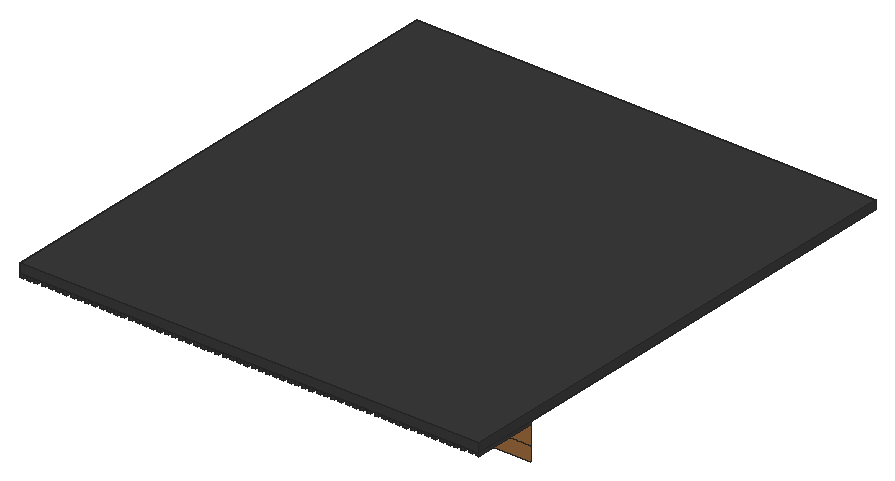
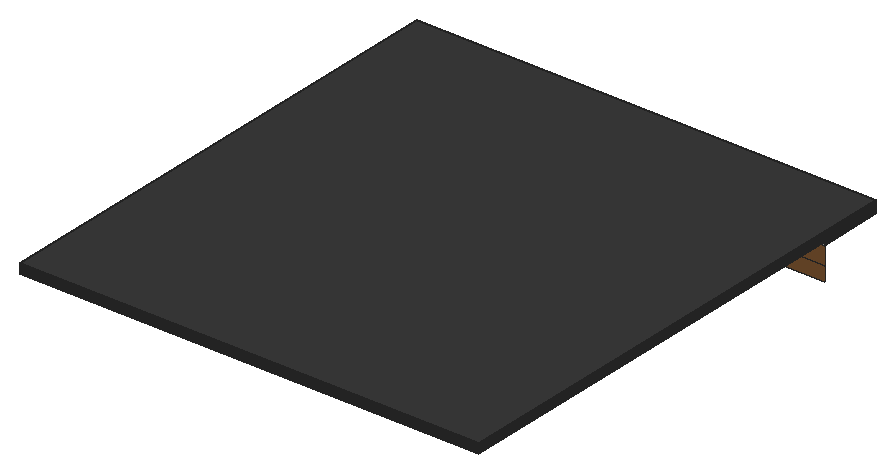
# SketchUp Ruby script. Lengths in inches.
U = 1.inch
M = Sketchup.active_model
def pt(a) = Geom::Point3d.new(a.map { |v| v * U })
def face(e, loops, mat)
  f = e.add_face(loops[0].map { |a| pt(a) })
  loops[1..].each { |l| e.add_face(l.map { |a| pt(a) }).erase! }
  f.material = f.back_material = mat if mat
  f
end
# faces: each face lists its corners as indices into pts; further lists are holes
def faces(e, pts, list, mat = nil) = list.each { |f| face(e, (f[0].is_a?(Array) ? f : [f]).map { |l| l.map { |i| pts[i] } }, mat) }
# xy, xz, yz: faces in a plane at the given z, y or x. An outline is a flat list of corners, or four numbers for a rectangle; further outlines are holes
def ring(l) = l.size == 4 ? [[l[0], l[1]], [l[2], l[1]], [l[2], l[3]], [l[0], l[3]]] : l.each_slice(2).to_a
def flat(e, list, mat, &to3) = list.each { |f| face(e, (f[0].is_a?(Array) ? f : [f]).map { |l| ring(l).map { |u, v| to3.(u, v) } }, mat) }
def xy(e, z, list, mat = nil) = flat(e, list, mat) { |x, y| [x, y, z] }
def xz(e, y, list, mat = nil) = flat(e, list, mat) { |x, z| [x, y, z] }
def yz(e, x, list, mat = nil) = flat(e, list, mat) { |y, z| [x, y, z] }
def lines(e, pts, list) = list.each { |a, b| e.add_line(pt(pts[a]), pt(pts[b])) }
# prism: a flat outline (further loops are holes) pulled along v
def prism(e, loops, v, mat = nil)
  f = face(e, loops, mat); d = Geom::Vector3d.new(v.map { |x| x * U })
  f.pushpull(f.normal.samedirection?(d) ? d.length : -d.length)
end
def box(e, o, s, mat = nil) = prism(e, [[o, [o[0] + s[0], o[1], o[2]], [o[0] + s[0], o[1] + s[1], o[2]], [o[0], o[1] + s[1], o[2]]]], [0, 0, s[2]], mat)
def at(x, y, z, deg = 0) = Geom::Transformation.translation(pt([x, y, z])) * Geom::Transformation.rotation(ORIGIN, Z_AXIS, deg.degrees)
def axes(o, x, y, z) = Geom::Transformation.new([*x, 0, *y, 0, *z, 0, *pt(o).to_a, 1])
def part(name) = M.definitions.add(name)
# library, detail: a bought-in or finely detailed component or shape, given as its bounding box
def library(name, o, s) = part(name).tap { |d| box(d.entities, o, s) }
def detail(e, o, s) = box(e.add_group.entities, o, s)
def put(e, d, t, mat = nil) = e.add_instance(d, t).tap { |i| i.material = mat if mat }
def group(e, t, mat = nil) = e.add_group.tap { |g| g.transformation = t; g.material = mat if mat }.entities
root = M.entities
M.materials.add("[Color M07]").color = [58, 58, 58]
M.materials.add("[Wood Floor]").color = [155, 105, 61]
xy(root,660.9375,[[24,175.75,456,528]])
xy(root,663.4375,[[0,33.5625,4.18,100.625],[7.5625,33.5625,11.74,100.625],[15.125,33.5625,19.31,100.625],[22.6875,33.5625,26.87,100.625],[30.25,33.5625,34.43,100.625],
  [37.8125,33.5625,41.99,100.625],[45.375,33.5625,49.56,100.625],[52.9375,33.5625,57.12,100.625],[60.5,33.5625,64.68,100.625],[68.0625,33.5625,72.24,100.625],
  [75.625,33.5625,79.81,100.625],[83.1875,33.5625,87.37,100.625],[90.75,33.5625,94.93,100.625],[98.3125,33.5625,102.49,100.625],[105.875,33.5625,110.06,100.625],
  [113.4375,33.5625,117.62,100.625],[121,33.5625,125.18,100.625],[128.5625,33.5625,132.74,100.625],[136.125,33.5625,140.31,100.625],[143.6875,33.5625,147.87,100.625],
  [151.25,33.5625,155.43,100.625],[158.8125,33.5625,162.99,100.625],[166.375,33.5625,170.56,100.625],[173.9375,33.5625,178.12,100.625],[181.5,33.5625,185.68,100.625],
  [189.0625,33.5625,193.24,100.625],[196.625,33.5625,200.81,100.625],[204.1875,33.5625,208.37,100.625],[211.75,33.5625,215.93,100.625],[219.3125,33.5625,223.49,100.625],
  [226.875,33.5625,231.06,100.625],[234.4375,33.5625,238.62,100.625],[242,33.5625,246.18,100.625],[249.5625,33.5625,253.74,100.625],[257.125,33.5625,261.31,100.625],
  [264.6875,33.5625,268.87,100.625],[272.25,33.5625,276.43,100.625],[279.8125,33.5625,283.99,100.625],[287.375,33.5625,291.56,100.625],[294.9375,33.5625,299.12,100.625],
  [302.5,33.5625,306.68,100.625],[310.0625,33.5625,314.24,100.625]],"[Color M07]")
xy(root,663.9,[[317.625,33.5625,321.81,100.625],[325.1875,33.5625,329.37,100.625],[332.75,33.5625,336.93,100.625],[340.3125,33.5625,344.49,100.625],[347.875,33.5625,352.06,100.625],
  [355.4375,33.5625,359.62,100.625],[363,33.5625,367.18,100.625],[370.5625,33.5625,374.74,100.625],[378.125,33.5625,382.31,100.625],[385.6875,33.5625,389.87,100.625],
  [393.25,33.5625,397.43,100.625],[400.8125,33.5625,404.99,100.625],[408.375,33.5625,412.56,100.625],[415.9375,33.5625,420.12,100.625],[423.5,33.5625,427.68,100.625],
  [431.0625,33.5625,435.24,100.625],[438.625,33.5625,442.81,100.625],[446.1875,33.5625,450.37,100.625],[453.75,33.5625,457.93,100.625],[461.3125,33.5625,465.49,100.625],
  [468.875,33.5625,473.06,100.625],[476.4375,33.5625,480,100.625]],"[Color M07]")
xy(root,666.9375,[[0,33.5625,4.18,100.625],[7.5625,33.5625,11.74,100.625],[15.125,33.5625,19.31,100.625],[22.6875,33.5625,26.87,100.625],[30.25,33.5625,34.43,100.625],
  [37.8125,33.5625,41.99,100.625],[45.375,33.5625,49.56,100.625],[52.9375,33.5625,57.12,100.625],[60.5,33.5625,64.68,100.625],[68.0625,33.5625,72.24,100.625],
  [75.625,33.5625,79.81,100.625],[83.1875,33.5625,87.37,100.625],[90.75,33.5625,94.93,100.625],[98.3125,33.5625,102.49,100.625],[105.875,33.5625,110.06,100.625],
  [113.4375,33.5625,117.62,100.625],[121,33.5625,125.18,100.625],[128.5625,33.5625,132.74,100.625],[136.125,33.5625,140.31,100.625],[143.6875,33.5625,147.87,100.625],
  [151.25,33.5625,155.43,100.625],[158.8125,33.5625,162.99,100.625],[166.375,33.5625,170.56,100.625],[173.9375,33.5625,178.12,100.625],[181.5,33.5625,185.68,100.625],
  [189.0625,33.5625,193.24,100.625],[196.625,33.5625,200.81,100.625],[204.1875,33.5625,208.37,100.625],[211.75,33.5625,215.93,100.625],[219.3125,33.5625,223.49,100.625],
  [226.875,33.5625,231.06,100.625],[234.4375,33.5625,238.62,100.625],[242,33.5625,246.18,100.625],[249.5625,33.5625,253.74,100.625],[257.125,33.5625,261.31,100.625],
  [264.6875,33.5625,268.87,100.625],[272.25,33.5625,276.43,100.625],[279.8125,33.5625,283.99,100.625],[287.375,33.5625,291.56,100.625],[294.9375,33.5625,299.12,100.625],
  [302.5,33.5625,306.68,100.625],[310.0625,33.5625,314.24,100.625],[317.625,33.5625,321.81,100.625],[325.1875,33.5625,329.37,100.625],[332.75,33.5625,336.93,100.625],
  [340.3125,33.5625,344.49,100.625],[347.875,33.5625,352.06,100.625],[355.4375,33.5625,359.62,100.625],[363,33.5625,367.18,100.625],[370.5625,33.5625,374.74,100.625],
  [378.125,33.5625,382.31,100.625],[385.6875,33.5625,389.87,100.625],[393.25,33.5625,397.43,100.625],[400.8125,33.5625,404.99,100.625],[408.375,33.5625,412.56,100.625],
  [415.9375,33.5625,420.12,100.625],[423.5,33.5625,427.68,100.625],[431.0625,33.5625,435.24,100.625],[438.625,33.5625,442.81,100.625],[446.1875,33.5625,450.37,100.625],
  [453.75,33.5625,457.93,100.625],[461.3125,33.5625,465.49,100.625],[468.875,33.5625,473.06,100.625],[476.4375,33.5625,480,100.625],[0,100.625,480,552]])
xy(root,666.9375,[[4.18,33.5625,7.5625,100.625],[11.74,33.5625,15.125,100.625],[19.31,33.5625,22.6875,100.625],[26.87,33.5625,30.25,100.625],[34.43,33.5625,37.8125,100.625],
  [41.99,33.5625,45.375,100.625],[49.56,33.5625,52.9375,100.625],[57.12,33.5625,60.5,100.625],[64.68,33.5625,68.0625,100.625],[72.24,33.5625,75.625,100.625],
  [79.81,33.5625,83.1875,100.625],[87.37,33.5625,90.75,100.625],[94.93,33.5625,98.3125,100.625],[102.49,33.5625,105.875,100.625],[110.06,33.5625,113.4375,100.625],
  [117.62,33.5625,121,100.625],[125.18,33.5625,128.5625,100.625],[132.74,33.5625,136.125,100.625],[140.31,33.5625,143.6875,100.625],[147.87,33.5625,151.25,100.625],
  [155.43,33.5625,158.8125,100.625],[162.99,33.5625,166.375,100.625],[170.56,33.5625,173.9375,100.625],[178.12,33.5625,181.5,100.625],[185.68,33.5625,189.0625,100.625],
  [193.24,33.5625,196.625,100.625],[200.81,33.5625,204.1875,100.625],[208.37,33.5625,211.75,100.625],[215.93,33.5625,219.3125,100.625],[223.49,33.5625,226.875,100.625],
  [231.06,33.5625,234.4375,100.625],[238.62,33.5625,242,100.625],[246.18,33.5625,249.5625,100.625],[253.74,33.5625,257.125,100.625],[261.31,33.5625,264.6875,100.625],
  [268.87,33.5625,272.25,100.625],[276.43,33.5625,279.8125,100.625],[283.99,33.5625,287.375,100.625],[291.56,33.5625,294.9375,100.625],[299.12,33.5625,302.5,100.625],
  [306.68,33.5625,310.0625,100.625],[314.24,33.5625,317.625,100.625],[321.81,33.5625,325.1875,100.625],[329.37,33.5625,332.75,100.625],[336.93,33.5625,340.3125,100.625],
  [344.49,33.5625,347.875,100.625],[352.06,33.5625,355.4375,100.625],[359.62,33.5625,363,100.625],[367.18,33.5625,370.5625,100.625],[374.74,33.5625,378.125,100.625],
  [382.31,33.5625,385.6875,100.625],[389.87,33.5625,393.25,100.625],[397.43,33.5625,400.8125,100.625],[404.99,33.5625,408.375,100.625],[412.56,33.5625,415.9375,100.625],
  [420.12,33.5625,423.5,100.625],[427.68,33.5625,431.0625,100.625],[435.24,33.5625,438.625,100.625],[442.81,33.5625,446.1875,100.625],[450.37,33.5625,453.75,100.625],
  [457.93,33.5625,461.3125,100.625],[465.49,33.5625,468.875,100.625],[473.06,33.5625,476.4375,100.625]],"[Color M07]")
xy(root,676.5625,[[0,33.5625,480,552]],"[Color M07]")
xz(root,33.5625,[[0,663.4375,4.18,666.9375],[7.5625,663.4375,11.74,666.9375],[15.125,663.4375,19.31,666.9375],[22.6875,663.4375,26.87,666.9375],[30.25,663.4375,34.43,666.9375],
  [37.8125,663.4375,41.99,666.9375],[45.375,663.4375,49.56,666.9375],[52.9375,663.4375,57.12,666.9375],[60.5,663.4375,64.68,666.9375],[68.0625,663.4375,72.24,666.9375],
  [75.625,663.4375,79.81,666.9375],[83.1875,663.4375,87.37,666.9375],[90.75,663.4375,94.93,666.9375],[98.3125,663.4375,102.49,666.9375],[105.875,663.4375,110.06,666.9375],
  [113.4375,663.4375,117.62,666.9375],[121,663.4375,125.18,666.9375],[128.5625,663.4375,132.74,666.9375],[136.125,663.4375,140.31,666.9375],[143.6875,663.4375,147.87,666.9375],
  [151.25,663.4375,155.43,666.9375],[158.8125,663.4375,162.99,666.9375],[166.375,663.4375,170.56,666.9375],[173.9375,663.4375,178.12,666.9375],[181.5,663.4375,185.68,666.9375],
  [189.0625,663.4375,193.24,666.9375],[196.625,663.4375,200.81,666.9375],[204.1875,663.4375,208.37,666.9375],[211.75,663.4375,215.93,666.9375],[219.3125,663.4375,223.49,666.9375],
  [226.875,663.4375,231.06,666.9375],[234.4375,663.4375,238.62,666.9375],[242,663.4375,246.18,666.9375],[249.5625,663.4375,253.74,666.9375],[257.125,663.4375,261.31,666.9375],
  [264.6875,663.4375,268.87,666.9375],[272.25,663.4375,276.43,666.9375],[279.8125,663.4375,283.99,666.9375],[287.375,663.4375,291.56,666.9375],[294.9375,663.4375,299.12,666.9375],
  [302.5,663.4375,306.68,666.9375],[310.0625,663.4375,314.24,666.9375],[317.625,663.9,321.81,666.9375],[325.1875,663.9,329.37,666.9375],[332.75,663.9,336.93,666.9375],
  [340.3125,663.9,344.49,666.9375],[347.875,663.9,352.06,666.9375],[355.4375,663.9,359.62,666.9375],[363,663.9,367.18,666.9375],[370.5625,663.9,374.74,666.9375],
  [378.125,663.9,382.31,666.9375],[385.6875,663.9,389.87,666.9375],[393.25,663.9,397.43,666.9375],[400.8125,663.9,404.99,666.9375],[408.375,663.9,412.56,666.9375],
  [415.9375,663.9,420.12,666.9375],[423.5,663.9,427.68,666.9375],[431.0625,663.9,435.24,666.9375],[438.625,663.9,442.81,666.9375],[446.1875,663.9,450.37,666.9375],
  [453.75,663.9,457.93,666.9375],[461.3125,663.9,465.49,666.9375],[468.875,663.9,473.06,666.9375],[476.4375,663.9,480,666.9375],[0,666.9375,480,676.5625]],"[Color M07]")
xz(root,100.625,[[0,663.4375,4.18,666.9375],[7.5625,663.4375,11.74,666.9375],[15.125,663.4375,19.31,666.9375],[22.6875,663.4375,24,666.9375],[24,663.4375,26.87,666.9375],
  [30.25,663.4375,34.43,666.9375],[37.8125,663.4375,41.99,666.9375],[45.375,663.4375,49.56,666.9375],[52.9375,663.4375,57.12,666.9375],[60.5,663.4375,64.68,666.9375],
  [68.0625,663.4375,72.24,666.9375],[75.625,663.4375,79.81,666.9375],[83.1875,663.4375,87.37,666.9375],[90.75,663.4375,94.93,666.9375],[98.3125,663.4375,102.49,666.9375],
  [105.875,663.4375,110.06,666.9375],[113.4375,663.4375,117.62,666.9375],[121,663.4375,125.18,666.9375],[128.5625,663.4375,132.74,666.9375],[136.125,663.4375,140.31,666.9375],
  [143.6875,663.4375,147.87,666.9375],[151.25,663.4375,155.43,666.9375],[158.8125,663.4375,162.99,666.9375],[166.375,663.4375,170.56,666.9375],[173.9375,663.4375,178.12,666.9375],
  [181.5,663.4375,185.68,666.9375],[189.0625,663.4375,193.24,666.9375],[196.625,663.4375,200.81,666.9375],[204.1875,663.4375,208.37,666.9375],[211.75,663.4375,215.93,666.9375],
  [219.3125,663.4375,223.49,666.9375],[226.875,663.4375,231.06,666.9375],[234.4375,663.4375,238.62,666.9375],[242,663.4375,246.18,666.9375],[249.5625,663.4375,253.74,666.9375],
  [257.125,663.4375,261.31,666.9375],[264.6875,663.4375,268.87,666.9375],[272.25,663.4375,276.43,666.9375],[279.8125,663.4375,283.99,666.9375],[287.375,663.4375,291.56,666.9375],
  [294.9375,663.4375,299.12,666.9375],[302.5,663.4375,306.68,666.9375],[310.0625,663.4375,314.24,666.9375],[317.625,663.9,321.81,666.9375],[325.1875,663.9,329.37,666.9375],
  [332.75,663.9,336.93,666.9375],[340.3125,663.9,344.49,666.9375],[347.875,663.9,352.06,666.9375],[355.4375,663.9,359.62,666.9375],[363,663.9,367.18,666.9375],
  [370.5625,663.9,374.74,666.9375],[378.125,663.9,382.31,666.9375],[385.6875,663.9,389.87,666.9375],[393.25,663.9,397.43,666.9375],[400.8125,663.9,404.99,666.9375],
  [408.375,663.9,412.56,666.9375],[415.9375,663.9,420.12,666.9375],[423.5,663.9,427.68,666.9375],[431.0625,663.9,435.24,666.9375],[438.625,663.9,442.81,666.9375],
  [446.1875,663.9,450.37,666.9375],[453.75,663.9,456,666.9375],[456,663.9,457.93,666.9375],[461.3125,663.9,465.49,666.9375],[468.875,663.9,473.06,666.9375],
  [476.4375,663.9,480,666.9375]])
xz(root,100.625,[[0,629.46,480,644.15],[0,644.15,480,644.15,480,663.9,476.4375,663.9,476.4375,666.9375,473.06,666.9375,473.06,663.9,468.875,663.9,468.875,666.9375,465.49,666.9375,465.49,663.9,461.3125,663.9,461.3125,666.9375,457.93,666.9375,457.93,663.9,453.75,663.9,453.75,666.9375,450.37,666.9375,450.37,663.9,446.1875,663.9,446.1875,666.9375,442.81,666.9375,442.81,663.9,438.625,663.9,438.625,666.9375,435.24,666.9375,435.24,663.9,431.0625,663.9,431.0625,666.9375,427.68,666.9375,427.68,663.9,423.5,663.9,423.5,666.9375,420.12,666.9375,420.12,663.9,415.9375,663.9,415.9375,666.9375,412.56,666.9375,412.56,663.9,408.375,663.9,408.375,666.9375,404.99,666.9375,404.99,663.9,400.8125,663.9,400.8125,666.9375,397.43,666.9375,397.43,663.9,393.25,663.9,393.25,666.9375,389.87,666.9375,389.87,663.9,385.6875,663.9,385.6875,666.9375,382.31,666.9375,382.31,663.9,378.125,663.9,378.125,666.9375,374.74,666.9375,374.74,663.9,370.5625,663.9,370.5625,666.9375,367.18,666.9375,367.18,663.9,363,663.9,363,666.9375,359.62,666.9375,359.62,663.9,355.4375,663.9,355.4375,666.9375,352.06,666.9375,352.06,663.9,347.875,663.9,347.875,666.9375,344.49,666.9375,344.49,663.9,340.3125,663.9,340.3125,666.9375,336.93,666.9375,336.93,663.9,332.75,663.9,332.75,666.9375,329.37,666.9375,329.37,663.9,325.1875,663.9,325.1875,666.9375,321.81,666.9375,321.81,663.9,317.625,663.9,317.625,666.9375,314.24,666.9375,314.24,663.4375,310.0625,663.4375,310.0625,666.9375,306.68,666.9375,306.68,663.4375,302.5,663.4375,302.5,666.9375,299.12,666.9375,299.12,663.4375,294.9375,663.4375,294.9375,666.9375,291.56,666.9375,291.56,663.4375,287.375,663.4375,287.375,666.9375,283.99,666.9375,283.99,663.4375,279.8125,663.4375,279.8125,666.9375,276.43,666.9375,276.43,663.4375,272.25,663.4375,272.25,666.9375,268.87,666.9375,268.87,663.4375,264.6875,663.4375,264.6875,666.9375,261.31,666.9375,261.31,663.4375,257.125,663.4375,257.125,666.9375,253.74,666.9375,253.74,663.4375,249.5625,663.4375,249.5625,666.9375,246.18,666.9375,246.18,663.4375,242,663.4375,242,666.9375,238.62,666.9375,238.62,663.4375,234.4375,663.4375,234.4375,666.9375,231.06,666.9375,231.06,663.4375,226.875,663.4375,226.875,666.9375,223.49,666.9375,223.49,663.4375,219.3125,663.4375,219.3125,666.9375,215.93,666.9375,215.93,663.4375,211.75,663.4375,211.75,666.9375,208.37,666.9375,208.37,663.4375,204.1875,663.4375,204.1875,666.9375,200.81,666.9375,200.81,663.4375,196.625,663.4375,196.625,666.9375,193.24,666.9375,193.24,663.4375,189.0625,663.4375,189.0625,666.9375,185.68,666.9375,185.68,663.4375,181.5,663.4375,181.5,666.9375,178.12,666.9375,178.12,663.4375,173.9375,663.4375,173.9375,666.9375,170.56,666.9375,170.56,663.4375,166.375,663.4375,166.375,666.9375,162.99,666.9375,162.99,663.4375,158.8125,663.4375,158.8125,666.9375,155.43,666.9375,155.43,663.4375,151.25,663.4375,151.25,666.9375,147.87,666.9375,147.87,663.4375,143.6875,663.4375,143.6875,666.9375,140.31,666.9375,140.31,663.4375,136.125,663.4375,136.125,666.9375,132.74,666.9375,132.74,663.4375,128.5625,663.4375,128.5625,666.9375,125.18,666.9375,125.18,663.4375,121,663.4375,121,666.9375,117.62,666.9375,117.62,663.4375,113.4375,663.4375,113.4375,666.9375,110.06,666.9375,110.06,663.4375,105.875,663.4375,105.875,666.9375,102.49,666.9375,102.49,663.4375,98.3125,663.4375,98.3125,666.9375,94.93,666.9375,94.93,663.4375,90.75,663.4375,90.75,666.9375,87.37,666.9375,87.37,663.4375,83.1875,663.4375,83.1875,666.9375,79.81,666.9375,79.81,663.4375,75.625,663.4375,75.625,666.9375,72.24,666.9375,72.24,663.4375,68.0625,663.4375,68.0625,666.9375,64.68,666.9375,64.68,663.4375,60.5,663.4375,60.5,666.9375,57.12,666.9375,57.12,663.4375,52.9375,663.4375,52.9375,666.9375,49.56,666.9375,49.56,663.4375,45.375,663.4375,45.375,666.9375,41.99,666.9375,41.99,663.4375,37.8125,663.4375,37.8125,666.9375,34.43,666.9375,34.43,663.4375,30.25,663.4375,30.25,666.9375,26.87,666.9375,26.87,663.4375,22.6875,663.4375,22.6875,666.9375,19.31,666.9375,19.31,663.4375,15.125,663.4375,15.125,666.9375,11.74,666.9375,11.74,663.4375,7.5625,663.4375,7.5625,666.9375,4.18,666.9375,4.18,663.4375,0,663.4375]],"[Wood Floor]")
xz(root,552,[[0,666.9375,480,676.5625]],"[Color M07]")
yz(root,0,[[33.5625,663.4375,100.625,666.9375],[33.5625,666.9375,552,676.5625]],"[Color M07]")
yz(root,4.18,[[33.5625,663.4375,100.625,666.9375]],"[Color M07]")
yz(root,7.5625,[[33.5625,663.4375,100.625,666.9375]],"[Color M07]")
yz(root,11.74,[[33.5625,663.4375,100.625,666.9375]],"[Color M07]")
yz(root,15.125,[[33.5625,663.4375,100.625,666.9375]],"[Color M07]")
yz(root,19.31,[[33.5625,663.4375,100.625,666.9375]],"[Color M07]")
yz(root,22.6875,[[33.5625,663.4375,100.625,666.9375]],"[Color M07]")
yz(root,26.87,[[33.5625,663.4375,100.625,666.9375]],"[Color M07]")
yz(root,30.25,[[33.5625,663.4375,100.625,666.9375]],"[Color M07]")
yz(root,34.43,[[33.5625,663.4375,100.625,666.9375]],"[Color M07]")
yz(root,37.8125,[[33.5625,663.4375,100.625,666.9375]],"[Color M07]")
yz(root,41.99,[[33.5625,663.4375,100.625,666.9375]],"[Color M07]")
yz(root,45.375,[[33.5625,663.4375,100.625,666.9375]],"[Color M07]")
yz(root,49.56,[[33.5625,663.4375,100.625,666.9375]],"[Color M07]")
yz(root,52.9375,[[33.5625,663.4375,100.625,666.9375]],"[Color M07]")
yz(root,57.12,[[33.5625,663.4375,100.625,666.9375]],"[Color M07]")
yz(root,60.5,[[33.5625,663.4375,100.625,666.9375]],"[Color M07]")
yz(root,64.68,[[33.5625,663.4375,100.625,666.9375]],"[Color M07]")
yz(root,68.0625,[[33.5625,663.4375,100.625,666.9375]],"[Color M07]")
yz(root,72.24,[[33.5625,663.4375,100.625,666.9375]],"[Color M07]")
yz(root,75.625,[[33.5625,663.4375,100.625,666.9375]],"[Color M07]")
yz(root,79.81,[[33.5625,663.4375,100.625,666.9375]],"[Color M07]")
yz(root,83.1875,[[33.5625,663.4375,100.625,666.9375]],"[Color M07]")
yz(root,87.37,[[33.5625,663.4375,100.625,666.9375]],"[Color M07]")
yz(root,90.75,[[33.5625,663.4375,100.625,666.9375]],"[Color M07]")
yz(root,94.93,[[33.5625,663.4375,100.625,666.9375]],"[Color M07]")
yz(root,98.3125,[[33.5625,663.4375,100.625,666.9375]],"[Color M07]")
yz(root,102.49,[[33.5625,663.4375,100.625,666.9375]],"[Color M07]")
yz(root,105.875,[[33.5625,663.4375,100.625,666.9375]],"[Color M07]")
yz(root,110.06,[[33.5625,663.4375,100.625,666.9375]],"[Color M07]")
yz(root,113.4375,[[33.5625,663.4375,100.625,666.9375]],"[Color M07]")
yz(root,117.62,[[33.5625,663.4375,100.625,666.9375]],"[Color M07]")
yz(root,121,[[33.5625,663.4375,100.625,666.9375]],"[Color M07]")
yz(root,125.18,[[33.5625,663.4375,100.625,666.9375]],"[Color M07]")
yz(root,128.5625,[[33.5625,663.4375,100.625,666.9375]],"[Color M07]")
yz(root,132.74,[[33.5625,663.4375,100.625,666.9375]],"[Color M07]")
yz(root,136.125,[[33.5625,663.4375,100.625,666.9375]],"[Color M07]")
yz(root,140.31,[[33.5625,663.4375,100.625,666.9375]],"[Color M07]")
yz(root,143.6875,[[33.5625,663.4375,100.625,666.9375]],"[Color M07]")
yz(root,147.87,[[33.5625,663.4375,100.625,666.9375]],"[Color M07]")
yz(root,151.25,[[33.5625,663.4375,100.625,666.9375]],"[Color M07]")
yz(root,155.43,[[33.5625,663.4375,100.625,666.9375]],"[Color M07]")
yz(root,158.8125,[[33.5625,663.4375,100.625,666.9375]],"[Color M07]")
yz(root,162.99,[[33.5625,663.4375,100.625,666.9375]],"[Color M07]")
yz(root,166.375,[[33.5625,663.4375,100.625,666.9375]],"[Color M07]")
yz(root,170.56,[[33.5625,663.4375,100.625,666.9375]],"[Color M07]")
yz(root,173.9375,[[33.5625,663.4375,100.625,666.9375]],"[Color M07]")
yz(root,178.12,[[33.5625,663.4375,100.625,666.9375]],"[Color M07]")
yz(root,181.5,[[33.5625,663.4375,100.625,666.9375]],"[Color M07]")
yz(root,185.68,[[33.5625,663.4375,100.625,666.9375]],"[Color M07]")
yz(root,189.0625,[[33.5625,663.4375,100.625,666.9375]],"[Color M07]")
yz(root,193.24,[[33.5625,663.4375,100.625,666.9375]],"[Color M07]")
yz(root,196.625,[[33.5625,663.4375,100.625,666.9375]],"[Color M07]")
yz(root,200.81,[[33.5625,663.4375,100.625,666.9375]],"[Color M07]")
yz(root,204.1875,[[33.5625,663.4375,100.625,666.9375]],"[Color M07]")
yz(root,208.37,[[33.5625,663.4375,100.625,666.9375]],"[Color M07]")
yz(root,211.75,[[33.5625,663.4375,100.625,666.9375]],"[Color M07]")
yz(root,215.93,[[33.5625,663.4375,100.625,666.9375]],"[Color M07]")
yz(root,219.3125,[[33.5625,663.4375,100.625,666.9375]],"[Color M07]")
yz(root,223.49,[[33.5625,663.4375,100.625,666.9375]],"[Color M07]")
yz(root,226.875,[[33.5625,663.4375,100.625,666.9375]],"[Color M07]")
yz(root,231.06,[[33.5625,663.4375,100.625,666.9375]],"[Color M07]")
yz(root,234.4375,[[33.5625,663.4375,100.625,666.9375]],"[Color M07]")
yz(root,238.62,[[33.5625,663.4375,100.625,666.9375]],"[Color M07]")
yz(root,242,[[33.5625,663.4375,100.625,666.9375]],"[Color M07]")
yz(root,246.18,[[33.5625,663.4375,100.625,666.9375]],"[Color M07]")
yz(root,249.5625,[[33.5625,663.4375,100.625,666.9375]],"[Color M07]")
yz(root,253.74,[[33.5625,663.4375,100.625,666.9375]],"[Color M07]")
yz(root,257.125,[[33.5625,663.4375,100.625,666.9375]],"[Color M07]")
yz(root,261.31,[[33.5625,663.4375,100.625,666.9375]],"[Color M07]")
yz(root,264.6875,[[33.5625,663.4375,100.625,666.9375]],"[Color M07]")
yz(root,268.87,[[33.5625,663.4375,100.625,666.9375]],"[Color M07]")
yz(root,272.25,[[33.5625,663.4375,100.625,666.9375]],"[Color M07]")
yz(root,276.43,[[33.5625,663.4375,100.625,666.9375]],"[Color M07]")
yz(root,279.8125,[[33.5625,663.4375,100.625,666.9375]],"[Color M07]")
yz(root,283.99,[[33.5625,663.4375,100.625,666.9375]],"[Color M07]")
yz(root,287.375,[[33.5625,663.4375,100.625,666.9375]],"[Color M07]")
yz(root,291.56,[[33.5625,663.4375,100.625,666.9375]],"[Color M07]")
yz(root,294.9375,[[33.5625,663.4375,100.625,666.9375]],"[Color M07]")
yz(root,299.12,[[33.5625,663.4375,100.625,666.9375]],"[Color M07]")
yz(root,302.5,[[33.5625,663.4375,100.625,666.9375]],"[Color M07]")
yz(root,306.68,[[33.5625,663.4375,100.625,666.9375]],"[Color M07]")
yz(root,310.0625,[[33.5625,663.4375,100.625,666.9375]],"[Color M07]")
yz(root,314.24,[[33.5625,663.4375,100.625,666.9375]],"[Color M07]")
yz(root,317.625,[[33.5625,663.9,100.625,666.9375]],"[Color M07]")
yz(root,321.81,[[33.5625,663.9,100.625,666.9375]],"[Color M07]")
yz(root,325.1875,[[33.5625,663.9,100.625,666.9375]],"[Color M07]")
yz(root,329.37,[[33.5625,663.9,100.625,666.9375]],"[Color M07]")
yz(root,332.75,[[33.5625,663.9,100.625,666.9375]],"[Color M07]")
yz(root,336.93,[[33.5625,663.9,100.625,666.9375]],"[Color M07]")
yz(root,340.3125,[[33.5625,663.9,100.625,666.9375]],"[Color M07]")
yz(root,344.49,[[33.5625,663.9,100.625,666.9375]],"[Color M07]")
yz(root,347.875,[[33.5625,663.9,100.625,666.9375]],"[Color M07]")
yz(root,352.06,[[33.5625,663.9,100.625,666.9375]],"[Color M07]")
yz(root,355.4375,[[33.5625,663.9,100.625,666.9375]],"[Color M07]")
yz(root,359.62,[[33.5625,663.9,100.625,666.9375]],"[Color M07]")
yz(root,363,[[33.5625,663.9,100.625,666.9375]],"[Color M07]")
yz(root,367.18,[[33.5625,663.9,100.625,666.9375]],"[Color M07]")
yz(root,370.5625,[[33.5625,663.9,100.625,666.9375]],"[Color M07]")
yz(root,374.74,[[33.5625,663.9,100.625,666.9375]],"[Color M07]")
yz(root,378.125,[[33.5625,663.9,100.625,666.9375]],"[Color M07]")
yz(root,382.31,[[33.5625,663.9,100.625,666.9375]],"[Color M07]")
yz(root,385.6875,[[33.5625,663.9,100.625,666.9375]],"[Color M07]")
yz(root,389.87,[[33.5625,663.9,100.625,666.9375]],"[Color M07]")
yz(root,393.25,[[33.5625,663.9,100.625,666.9375]],"[Color M07]")
yz(root,397.43,[[33.5625,663.9,100.625,666.9375]],"[Color M07]")
yz(root,400.8125,[[33.5625,663.9,100.625,666.9375]],"[Color M07]")
yz(root,404.99,[[33.5625,663.9,100.625,666.9375]],"[Color M07]")
yz(root,408.375,[[33.5625,663.9,100.625,666.9375]],"[Color M07]")
yz(root,412.56,[[33.5625,663.9,100.625,666.9375]],"[Color M07]")
yz(root,415.9375,[[33.5625,663.9,100.625,666.9375]],"[Color M07]")
yz(root,420.12,[[33.5625,663.9,100.625,666.9375]],"[Color M07]")
yz(root,423.5,[[33.5625,663.9,100.625,666.9375]],"[Color M07]")
yz(root,427.68,[[33.5625,663.9,100.625,666.9375]],"[Color M07]")
yz(root,431.0625,[[33.5625,663.9,100.625,666.9375]],"[Color M07]")
yz(root,435.24,[[33.5625,663.9,100.625,666.9375]],"[Color M07]")
yz(root,438.625,[[33.5625,663.9,100.625,666.9375]],"[Color M07]")
yz(root,442.81,[[33.5625,663.9,100.625,666.9375]],"[Color M07]")
yz(root,446.1875,[[33.5625,663.9,100.625,666.9375]],"[Color M07]")
yz(root,450.37,[[33.5625,663.9,100.625,666.9375]],"[Color M07]")
yz(root,453.75,[[33.5625,663.9,100.625,666.9375]],"[Color M07]")
yz(root,457.93,[[33.5625,663.9,100.625,666.9375]],"[Color M07]")
yz(root,461.3125,[[33.5625,663.9,100.625,666.9375]],"[Color M07]")
yz(root,465.49,[[33.5625,663.9,100.625,666.9375]],"[Color M07]")
yz(root,468.875,[[33.5625,663.9,100.625,666.9375]],"[Color M07]")
yz(root,473.06,[[33.5625,663.9,100.625,666.9375]],"[Color M07]")
yz(root,476.4375,[[33.5625,663.9,100.625,666.9375]],"[Color M07]")
yz(root,480,[[33.5625,663.9,100.625,666.9375],[33.5625,666.9375,552,676.5625]],"[Color M07]")
p = [[40.625,528,666.9375],[40.625,528,660.9375],[24,175.75,660.9375],[24,175.75,666.9375],[456,175.75,660.9375],[456,175.75,666.9375]]
lines(root,p,[[0,1],[2,3],[4,5]])
